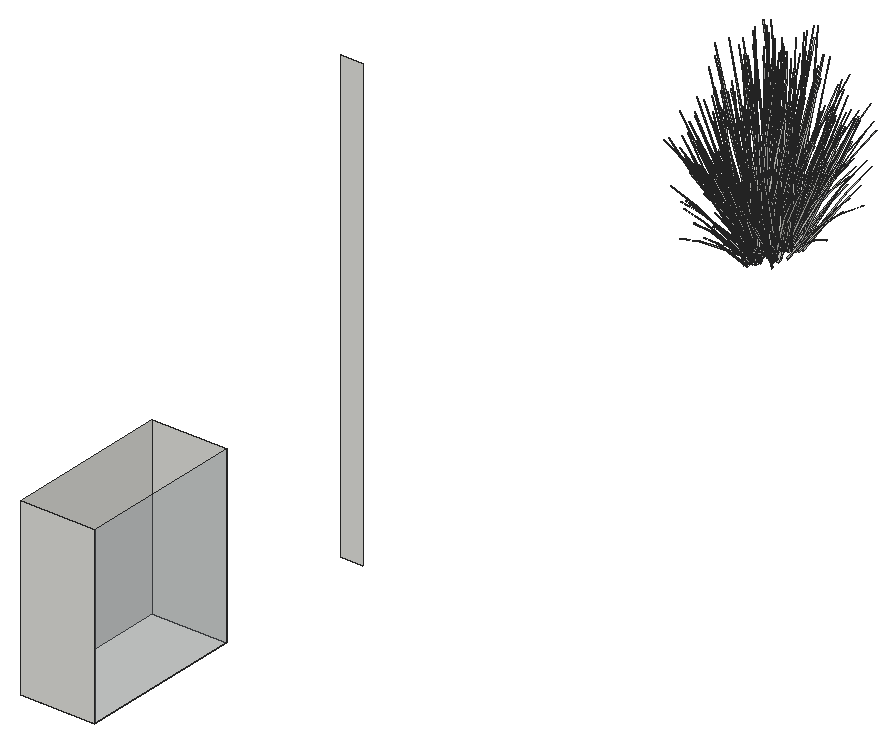
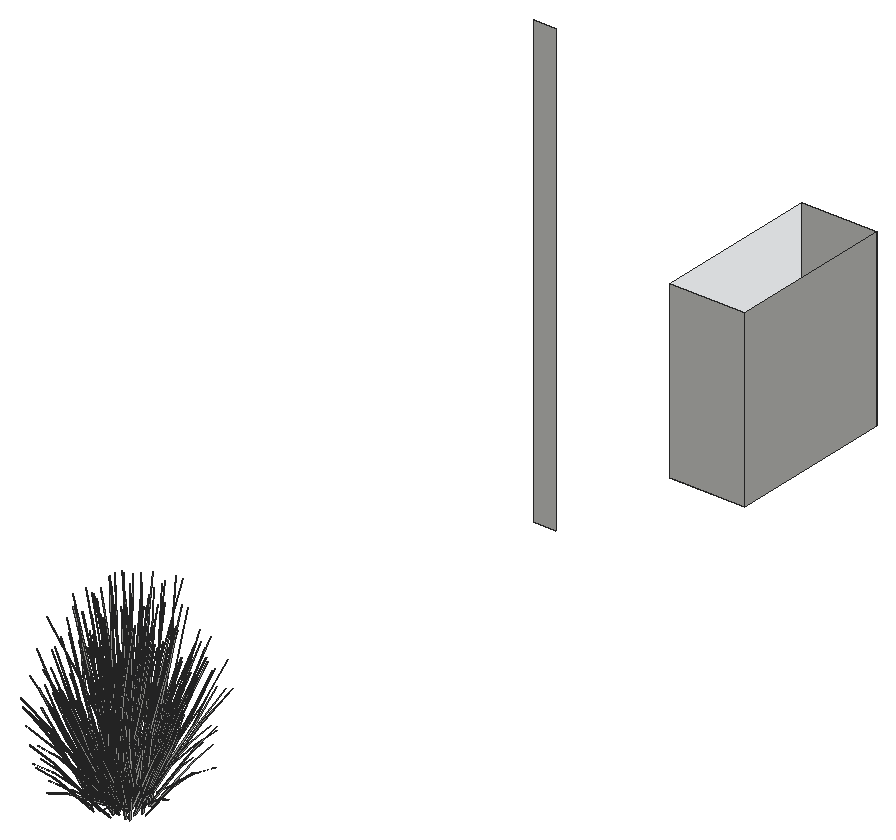
# SketchUp Ruby script. Lengths in inches.
U = 1.inch
M = Sketchup.active_model
def pt(a) = Geom::Point3d.new(a.map { |v| v * U })
def face(e, loops, mat)
  f = e.add_face(loops[0].map { |a| pt(a) })
  loops[1..].each { |l| e.add_face(l.map { |a| pt(a) }).erase! }
  f.material = f.back_material = mat if mat
  f
end
# faces: each face lists its corners as indices into pts; further lists are holes
def faces(e, pts, list, mat = nil) = list.each { |f| face(e, (f[0].is_a?(Array) ? f : [f]).map { |l| l.map { |i| pts[i] } }, mat) }
# xy, xz, yz: faces in a plane at the given z, y or x. An outline is a flat list of corners, or four numbers for a rectangle; further outlines are holes
def ring(l) = l.size == 4 ? [[l[0], l[1]], [l[2], l[1]], [l[2], l[3]], [l[0], l[3]]] : l.each_slice(2).to_a
def flat(e, list, mat, &to3) = list.each { |f| face(e, (f[0].is_a?(Array) ? f : [f]).map { |l| ring(l).map { |u, v| to3.(u, v) } }, mat) }
def xy(e, z, list, mat = nil) = flat(e, list, mat) { |x, y| [x, y, z] }
def xz(e, y, list, mat = nil) = flat(e, list, mat) { |x, z| [x, y, z] }
def yz(e, x, list, mat = nil) = flat(e, list, mat) { |y, z| [x, y, z] }
def lines(e, pts, list) = list.each { |a, b| e.add_line(pt(pts[a]), pt(pts[b])) }
# prism: a flat outline (further loops are holes) pulled along v
def prism(e, loops, v, mat = nil)
  f = face(e, loops, mat); d = Geom::Vector3d.new(v.map { |x| x * U })
  f.pushpull(f.normal.samedirection?(d) ? d.length : -d.length)
end
def box(e, o, s, mat = nil) = prism(e, [[o, [o[0] + s[0], o[1], o[2]], [o[0] + s[0], o[1] + s[1], o[2]], [o[0], o[1] + s[1], o[2]]]], [0, 0, s[2]], mat)
def at(x, y, z, deg = 0) = Geom::Transformation.translation(pt([x, y, z])) * Geom::Transformation.rotation(ORIGIN, Z_AXIS, deg.degrees)
def axes(o, x, y, z) = Geom::Transformation.new([*x, 0, *y, 0, *z, 0, *pt(o).to_a, 1])
def part(name) = M.definitions.add(name)
# library, detail: a bought-in or finely detailed component or shape, given as its bounding box
def library(name, o, s) = part(name).tap { |d| box(d.entities, o, s) }
def detail(e, o, s) = box(e.add_group.entities, o, s)
def put(e, d, t, mat = nil) = e.add_instance(d, t).tap { |i| i.material = mat if mat }
def group(e, t, mat = nil) = e.add_group.tap { |g| g.transformation = t; g.material = mat if mat }.entities
root = M.entities
M.materials.add("Glass_Basic_01").color = [161, 173, 186]
M.materials["Glass_Basic_01"].alpha = 0.25
c1 = part("blade")
p = [[2.15,0.21,22],[0,0.17,0],[0.09,0.45,0],[2.18,0.31,22],[2.29,0.31,22],[0.38,0.45,0],
  [2.48,0.24,33],[2.49,0.24,33],[2.48,0.22,33]]
faces(c1.entities,p,[[0,1,2,3],[4,5,2,3],[6,3,4,7],[8,0,3,6]])
c2 = part("blade with seeds\#1")
put(c2.entities,c1,at(0,0,0))
xy(root,122,[[460.07,50,480,94]])
xz(root,50,[[460.07,122,480,168.38]])
xz(root,94,[[460.07,122,480,168.38]])
xz(root,132,[[480,126,486,246]])
yz(root,460.07,[[50,122,94,168.38]])
yz(root,480,[[50,122,94,168.38]],"Glass_Basic_01")
put(root,c2,axes([472.34,285.93,129.63],[-1.0019,0.47479,-0.62955],[-0.36083,-1.36768,-0.16523],[-0.33927,0.05248,1.38963]))
put(root,c2,axes([474.05,281.59,129.625],[0.89455,-0.42392,-0.62393],[0.32217,1.22114,-0.16376],[0.30292,-0.04686,1.37722]))
put(root,c2,axes([472.17,281.71,129.59],[0.16018,-1.20264,-0.5621],[0.98808,0.25378,-0.14753],[0.11973,-0.3589,1.24074]))
put(root,c2,axes([474.21,285.74,129.59],[-0.16018,1.20264,-0.5621],[-0.98808,-0.25378,-0.14753],[-0.11973,0.3589,1.24074]))
put(root,c2,axes([471.31,283.85,129.59],[-0.73437,-0.77871,-0.5621],[0.66591,-0.96736,-0.14753],[-0.18319,-0.31204,1.24074]))
put(root,c2,axes([475.07,283.6,129.59],[0.73437,0.77871,-0.5621],[-0.66591,0.96736,-0.14753],[0.18319,0.31204,1.24074]))
put(root,c2,axes([470.3,280.13,129.56],[0.48852,-1.08202,-0.44759],[0.87598,0.64674,0],[0.11126,-0.24644,1.41987]))
put(root,c2,axes([477.07,282.32,129.56],[0.48852,1.08202,-0.44759],[-0.87598,0.64674,0],[0.11126,0.24644,1.41987]))
put(root,c2,axes([472.2,288.72,129.56],[-0.97703,0,-0.44759],[0,-1.29348,0],[-0.22253,0,1.41987]))
put(root,c2,axes([476.08,287.32,129.56],[-0.48852,1.08202,-0.44759],[-0.87598,-0.64674,0],[-0.11126,0.24644,1.41987]))
put(root,c2,axes([469.3125,285.13,129.56],[-0.48852,-1.08202,-0.44759],[0.87598,-0.64674,0],[-0.11126,-0.24644,1.41987]))
put(root,c2,axes([474.18,278.72,129.56],[0.97703,0,-0.44759],[0,1.29348,0],[0.22253,0,1.41987]))
put(root,c2,axes([472.6,285.2,129.73],[-0.88038,-0.56093,-0.40331],[0.4237,-1.16553,0.1941],[-0.20294,0,1.29492]))
put(root,c2,axes([473.9,285.12,129.73],[-0.82007,0.69452,-0.40331],[-0.57748,-1.05199,0.1941],[-0.10147,0.22475,1.29492]))
put(root,c2,axes([472.48,282.33,129.73],[0.82007,-0.69452,-0.40331],[0.57748,1.05199,0.1941],[0.10147,-0.22475,1.29492]))
put(root,c2,axes([473.78,282.25,129.73],[0.88038,0.56093,-0.40331],[-0.4237,1.16553,0.1941],[0.20294,0,1.29492]))
put(root,c2,axes([474.49,283.64,129.73],[0.06031,1.25545,-0.40331],[-1.00118,0.11354,0.1941],[0.10147,0.22475,1.29492]))
put(root,c2,axes([469.7,284.88,129.57],[0.24175,-1.0786,-0.27926],[0.85134,0.27158,0.27926],[-0.09817,-0.21744,1.25283]))
put(root,c2,axes([474.16,279.28,129.57],[0.60959,0.80703,-0.27926],[-0.60959,0.80703,0.27926],[0.19635,0,1.25283]))
put(root,c2,axes([475.72,287.02,129.57],[-0.85134,0.27158,-0.27926],[-0.24175,-1.0786,0.27926],[-0.09817,0.21744,1.25283]))
put(root,c2,axes([476.68,282.57,129.57],[-0.24175,1.0786,-0.27926],[-0.85134,-0.27158,0.27926],[0.09817,0.21744,1.25283]))
put(root,c2,axes([470.66,280.43,129.57],[0.85134,-0.27158,-0.27926],[0.24175,1.0786,0.27926],[0.09817,-0.21744,1.25283]))
put(root,c2,axes([472.22,288.17,129.57],[-0.60959,-0.80703,-0.27926],[0.60959,-0.80703,0.27926],[-0.19635,0,1.25283]))
put(root,c2,axes([477.25,280.18,129.08],[-0.14106,-0.08423,1.5897],[-0.41543,-1.06044,-0.24285],[0.21501,-0.3215,0.27078]))
put(root,c2,axes([472.82,289.61,129.08],[0.15398,-0.02932,1.5897],[0.80412,0.59108,-0.24285],[-0.04053,0.41985,0.27078]))
put(root,c2,axes([467.6,284.33,129.08],[0.0352,0.19392,1.5897],[-0.39624,1.07238,-0.24285],[-0.33051,-0.01799,0.27078]))
put(root,c2,axes([477.22,285.14,129.08],[-0.05317,-0.18711,1.5897],[0.29263,-1.12549,-0.24285],[0.32981,-0.03291,0.27078]))
put(root,c2,axes([472.97,277.13,129.08],[-0.14833,0.06042,1.5897],[-0.86768,-0.41907,-0.24285],[-0.01248,-0.42273,0.27078]))
put(root,c2,axes([468.81,287.79,129.08],[0.12871,0.11199,1.5897],[0.2775,1.13173,-0.24285],[-0.25244,0.2734,0.27078]))
put(root,c2,axes([477.13,289.92,129.08],[0.09761,-0.15508,1.5897],[0.90442,-0.26295,-0.24285],[0.19286,0.3437,0.27078]))
put(root,c2,axes([469.28,279.58,129.08],[-0.07697,0.17304,1.5897],[-0.85991,0.44448,-0.24285],[-0.23336,-0.29985,0.27078]))
put(root,c2,axes([471.44,286.02,129.17],[0.39117,1.13797,1.16227],[-1.12236,0.3622,0.45161],[0.01867,-0.69878,1.32195]))
put(root,c2,axes([475.32,282.36,129.71],[-0.33151,-1.21377,-0.17307],[0.95493,-0.4265,0.00007],[-0.03664,-0.13398,1.56765]))
put(root,c2,axes([474.22,282.76,130.14],[1.11485,-0.13472,-0.26229],[0.06741,1.40314,-0.45076],[0.1485,0.24708,1.43974]))
put(root,c2,axes([473.05,282.11,130.14],[0.46619,-1.302,-0.26229],[0.98396,0.62692,-0.45076],[0.24158,-0.04092,1.43974]))
put(root,c2,axes([473.33,285.34,130.14],[-0.46619,1.302,-0.26229],[-0.98396,-0.62692,-0.45076],[-0.24158,0.04092,1.43974]))
put(root,c2,axes([472.17,284.69,130.14],[-1.11485,0.13472,-0.26229],[-0.06741,-1.40314,-0.45076],[-0.1485,-0.24708,1.43974]))
put(root,c2,axes([472.02,283.07,130.14],[-0.64866,-1.16728,-0.26229],[0.91655,-0.77622,-0.45076],[0.09308,-0.288,1.43974]))
put(root,c2,axes([474.36,284.375,130.14],[0.64866,1.16728,-0.26229],[-0.91655,0.77622,-0.45076],[-0.09308,0.288,1.43974]))
put(root,c2,axes([474.65,283.07,129.96],[-0.78639,1.12892,-0.2271],[-0.88305,-0.94994,0.49699],[0.09199,0.304,1.51643]))
put(root,c2,axes([474.37,285.02,129.94],[-1.15773,-0.30643,-0.21121],[0.20181,-1.4529,0.4622],[-0.15988,0.25387,1.41028]))
put(root,c2,axes([468.28,284.53,129.65],[0.56051,0.79893,-0.03509],[-0.61388,0.73204,-0.15911],[-0.17394,0.05154,0.52479]))
put(root,c2,axes([469.3,288.5,129.65],[0.7978,0.33351,-0.03509],[-0.24541,1.02647,-0.15911],[-0.13049,0.15585,0.52479]))
put(root,c2,axes([472.75,276.59,129.77],[-0.62476,0.71677,-0.05849],[-0.57245,-0.78502,-0.26518],[-0.0403,-0.22243,0.87466]))
put(root,c2,axes([473.58,277.94,129.52],[0.11725,0.74462,1.27635],[-0.9333,0.11852,0.07306],[-0.14126,-0.52153,0.72629]))
put(root,c2,axes([469.46,286.11,129.875],[-0.97904,0.72283,0],[-0.54599,-1.20931,-0.46523],[-0.12435,-0.27543,1.47583]))
put(root,c2,axes([476.67,286.66,129.875],[0.97904,0.72283,0],[-0.54599,1.20931,-0.46523],[-0.12435,0.27543,1.47583]))
put(root,c2,axes([476.92,281.34,129.875],[0.97904,-0.72283,0],[0.54599,1.20931,-0.46523],[0.12435,0.27543,1.47583]))
put(root,c2,axes([472.94,289.05,129.875],[0,1.44565,0],[-1.09198,0,-0.46523],[-0.24871,0,1.47583]))
put(root,c2,axes([475.47,283.13,129.8],[1.12244,-0.50265,-0.0542],[0.39331,1.43622,0],[0.0392,-0.01755,1.55211]))
put(root,c2,axes([469.71,280.79,129.88],[-0.97904,-0.72283,0],[0.54599,-1.20931,-0.46523],[0.12435,-0.27543,1.47583]))
put(root,c2,axes([473.4375,278.4,129.88],[0,-1.44565,0],[1.09198,0,-0.46523],[0.24871,0,1.47583]))
put(root,c2,axes([473.71,282.8,129.81],[-0.84094,1.07538,-0.05527],[-0.84146,-1.07603,0],[-0.02937,0.03755,1.58274]))
put(root,c2,axes([473.28,282.4375,129.8],[1.12994,0,-0.05082],[0,1.44565,0],[0.03551,0,1.61697]))
put(root,c2,axes([476.81,282.25,129.71],[-0.98246,0.71382,-0.04636],[-0.54599,-1.20931,0.46523],[0.09354,0.298,1.4751]))
put(root,c2,axes([474,278.98,129.72],[-0.00781,1.44494,-0.04486],[-1.09198,0,0.45022],[0.24858,0.04541,1.42752]))
put(root,c2,axes([472.66,287.93,129.84],[0.82143,1.07538,0.27726],[-0.81279,1.07603,-0.32897],[-0.23327,0.03755,1.48641]))
put(root,c2,axes([476.3,282.22,129.84],[0.31757,-1.44738,0.27726],[1.13512,0.3621,-0.32897],[0.14207,0.23956,1.48641]))
put(root,c2,axes([475.82,284.03,129.72],[-0.43865,1.16553,0],[-0.91144,-0.56093,0],[0,0,1.46678]))
put(root,c2,axes([475.44,283.77,129.72],[-0.84234,0.37722,0],[-0.29498,-1.07717,0],[0,0,1.39163]))
put(root,c2,axes([475.84,282.71,129.72],[0.43865,-1.16553,0],[0.91144,0.56093,0],[0,0,1.57718]))
put(root,c2,axes([472.83,283.17,129.72],[-1.1305,0,0],[0,-1.44565,0],[0,0,1.61777]))
put(root,c2,axes([473.09,282.18,129.73],[0,-1.29348,0],[1.0115,0,0],[0,0,1.60831]))
put(root,c2,axes([473.52,282.21,129.73],[0.63109,-0.80703,0],[0.63109,0.80703,0],[0,0,1.52591]))
put(root,c2,axes([473.8125,284.85,129.87],[0.20585,-1.46124,0.41247],[1.16261,0.29738,0.16186],[-0.11226,0.21355,1.43206]))
put(root,c2,axes([472.12,283.85,129.87],[0.88667,0.95859,0.41247],[-0.7827,1.13884,0.16186],[-0.08849,-0.2311,1.43206]))
put(root,c2,axes([472.74,284.97,129.87],[1.09253,-0.50265,0.41247],[0.37991,1.43622,0.16186],[-0.20075,-0.01755,1.43206]))
put(root,c2,axes([472.57,282.6,129.88],[-0.20585,1.46124,0.44352],[-1.16261,-0.29738,0.17404],[0.11226,-0.21355,1.53985]))
put(root,c2,axes([474.43,282.5,130.1],[0.58702,-0.85413,0.13053],[0.66228,0.71246,-0.37274],[0.08953,0.19831,1.14258]))
put(root,c2,axes([471.74,282.96,130.1],[-0.87196,-0.22303,0.13053],[0.15136,-1.08968,-0.37274],[0.08953,-0.19831,1.14258]))
put(root,c2,axes([472.98,281.74,130.1],[-0.28493,-1.07717,0.13053],[0.81364,-0.37722,-0.37274],[0.17907,0,1.14258]))
put(root,c2,axes([474.64,284.49,130.1],[0.87196,0.22303,0.13053],[-0.15136,1.08968,-0.37274],[-0.08953,0.19831,1.14258]))
put(root,c2,axes([477.35,287.72,130.28],[-0.17302,-1.05027,0.05866],[0.69705,-0.24145,-0.77802],[0.35285,0.06658,0.69739]))
put(root,c2,axes([470.99,288.8,130.07],[0.27202,-0.22572,1.28914],[0.7394,0.52014,-0.27724],[-0.17673,0.53408,0.55117]))
put(root,c2,axes([478.09,287.98,130.07],[-0.15413,-0.36483,1.28914],[0.46474,-0.90077,-0.27724],[0.40213,0.2681,0.55117]))
put(root,c2,axes([475.91,282.68,130.07],[-0.32388,-0.0204,1.28914],[-0.36177,-0.97496,-0.27724],[0.38765,-0.30097,0.55117]))
put(root,c2,axes([468.67,281.875,130.07],[0.19776,0.32863,1.28914],[-0.34614,0.98419,-0.27724],[-0.43048,-0.18244,0.55117]))
put(root,c2,axes([471,278.71,130.07],[-0.02894,0.41302,1.28914],[-0.77632,0.42312,-0.27724],[-0.21961,-0.50739,0.55117]))
put(root,c2,axes([468.3,286.96,130.07],[0.31962,0.07001,1.28914],[0.26756,1.02347,-0.27724],[-0.41311,0.23924,0.55117]))
put(root,c2,axes([474.96,277.73,130.07],[-0.2403,0.27843,1.28914],[-0.79492,-0.36227,-0.27724],[0.10768,-0.56334,0.55117]))
put(root,c2,axes([474.96,290.35,130.07],[0.08021,-0.40179,1.28914],[0.81924,-0.25896,-0.27724],[0.15335,0.54576,0.55117]))
put(root,c2,axes([473.11,288.17,129.97],[0.97703,0,0.44759],[0,1.29348,0],[-0.22253,0,1.41987]))
put(root,c2,axes([470.22,281.41,129.97],[-0.48852,1.08202,0.44759],[-0.87598,-0.64674,0],[0.11126,-0.24644,1.41987]))
put(root,c2,axes([473.27,279.28,129.97],[-0.97703,0,0.44759],[0,-1.29348,0],[0.22253,0,1.41987]))
put(root,c2,axes([476.24,281.59,129.97],[-0.48852,-1.08202,0.44759],[0.87598,-0.64674,0],[0.11126,0.24644,1.41987]))
put(root,c2,axes([476.16,286.04,129.97],[0.48852,-1.08202,0.44759],[0.87598,0.64674,0],[-0.11126,0.24644,1.41987]))
put(root,c2,axes([473.04,284.51,129.93],[0.47355,-1.30265,0.21694],[0.98396,0.62692,0.45076],[-0.22682,0,1.44726]))
put(root,c2,axes([470.71,281.82,129.97],[0.25932,1.24233,0.15904],[-0.96507,0.30677,0.3163],[0.14061,-0.1108,1.44604]))
put(root,c2,axes([473.24,280.03,129.97],[-0.71168,0.90835,0.15904],[-0.69029,-0.91538,0.3163],[0.14534,0.10032,1.44604]))
put(root,c2,axes([470.66,285.51,129.97],[0.971,0.33398,0.15904],[-0.27478,1.22215,0.3163],[-0.00473,-0.21112,1.44604]))
put(root,c2,axes([475.72,281.94,129.97],[-0.971,-0.33398,0.15904],[0.27478,-1.22215,0.3163],[0.00473,0.21112,1.44604]))
put(root,c2,axes([475.67,285.63,129.97],[-0.25932,-1.24233,0.15904],[0.96507,-0.30677,0.3163],[-0.14061,0.1108,1.44604]))
put(root,c2,axes([472.78,282.22,130.1875],[-0.88038,-0.56093,0.40331],[0.4237,-1.16553,-0.1941],[0.20294,0,1.29492]))
put(root,c2,axes([472.38,284.93,130.1875],[0.06031,1.25545,0.40331],[-1.00118,0.11354,-0.1941],[-0.10147,-0.22475,1.29492]))
put(root,c2,axes([471.97,283.43,130.1875],[-0.82007,0.69452,0.40331],[-0.57748,-1.05199,-0.1941],[0.10147,-0.22475,1.29492]))
put(root,c2,axes([473.6,285.23,130.1875],[0.88038,0.56093,0.40331],[-0.4237,1.16553,-0.1941],[-0.20294,0,1.29492]))
put(root,c2,axes([474,282.52,130.1875],[-0.06031,-1.25545,0.40331],[1.00118,-0.11354,-0.1941],[0.10147,0.22475,1.29492]))
put(root,c2,axes([477.48,280.26,130.14],[-0.03064,0.74138,0.9471],[-0.6508,-0.48961,0.52291],[0.23122,-0.29288,0.74292]))
put(root,c2,axes([471.81,290.15,130.23],[-0.06991,-0.73811,1.03545],[0.616,0.4682,0.76078],[-0.09241,0.36475,0.22807]))
put(root,c2,axes([476.21,280.37,130.23],[-0.28093,0.65095,1.03545],[-0.28545,-0.84053,0.76078],[0.2418,-0.22671,0.22807]))
put(root,c2,axes([476.67,291.19,130.23],[-0.44281,-0.48182,1.03545],[0.70101,-0.19012,0.76078],[0.12552,0.34819,0.22807]))
put(root,c2,axes([473.9,276.4,130.23],[0.1613,0.71432,1.03545],[-0.66662,-0.33623,0.76078],[0.04561,-0.37895,0.22807]))
put(root,c2,axes([467.78,287.32,130.23],[0.34005,-0.60308,1.03545],[0.20441,0.87829,0.76078],[-0.26134,0.18792,0.22807]))
put(root,c2,axes([478.61,287.11,130.23],[-0.58095,0.02992,1.03545],[0.41436,-0.74764,0.76078],[0.2769,0.14704,0.22807]))
put(root,c2,axes([469.57,278.23,130.23],[0.49736,0.38508,1.03545],[-0.66822,0.331,0.76078],[-0.16744,-0.31805,0.22807]))
put(root,c2,axes([467.1,283.09,130.23],[0.56973,-0.14831,1.03545],[-0.31555,0.82274,0.76078],[-0.29172,-0.08853,0.22807]))
put(root,c2,axes([473.04,281.95,130.3],[-0.91991,0.03158,1.27354],[0.23846,-1.42935,0.53923],[0.50337,0.33806,1.20213]))
put(root,c2,axes([469.58,285.86,132.23],[-0.47225,0.98582,-0.64046],[-0.82754,-0.7006,0.07729],[-0.28197,0.35717,0.906]))
put(root,c2,axes([476.84,284.79,132.23],[0.79444,-0.5518,-0.64046],[0.44274,1.13586,0.07729],[0.38385,-0.12903,0.906]))
put(root,c2,axes([470.75,287.87,132.23],[-0.02352,1.1557,-0.64046],[-0.99061,-0.07762,0.07729],[-0.10454,0.48961,0.906]))
put(root,c2,axes([471.71,279.58,132.23],[-0.77091,-0.6039,-0.64046],[0.54787,-1.05824,0.07729],[-0.27931,-0.36058,0.906]))
put(root,c2,axes([473.65,279.3,132.23],[-0.4315,-1.0159,-0.64046],[0.88824,-0.56616,0.07729],[-0.1009,-0.49086,0.906]))
put(root,c2,axes([470.14,281.08,132.23],[-0.90375,-0.03008,-0.64046],[0.0607,-1.26677,0.07729],[-0.38287,-0.13368,0.906]))
put(root,c2,axes([475.45,280.29,132.23],[0.02352,-1.1557,-0.64046],[0.99061,0.07762,0.07729],[0.10454,-0.48961,0.906]))
put(root,c2,axes([469.36,283.375,132.23],[-0.79444,0.5518,-0.64046],[-0.44274,-1.13586,0.07729],[-0.38385,0.12903,0.906]))
put(root,c2,axes([477,284.37,131.96],[0.24493,-1.13649,-0.46065],[0.83975,0.38955,-0.35681],[0.33809,-0.10421,0.88141]))
put(root,c2,axes([469.84,281.33,131.96],[-0.65648,0.82762,-0.46065],[-0.57493,-0.87428,-0.35681],[-0.33354,-0.12593,0.88141]))
put(root,c2,axes([469.61,286.32,131.96],[0.23225,1.14083,-0.46065],[-0.87956,0.19957,-0.35681],[-0.25205,0.30642,0.88141]))
put(root,c2,axes([473.33,279.09,131.96],[-0.88873,-0.31321,-0.46065],[0.30463,-1.07385,-0.35681],[-0.08149,-0.43235,0.88141]))
put(root,c2,axes([470.95,288.25,131.96],[0.6472,0.83949,-0.46065],[-0.68369,0.73521,-0.35681],[-0.09847,0.42653,0.88141]))
put(root,c2,axes([474.85,288.55,131.96],[0.89213,-0.297,-0.46065],[0.15606,1.12475,-0.35681],[0.23962,0.32232,0.88141]))
put(root,c2,axes([472.87,289.07,131.96],[0.88873,0.31321,-0.46065],[-0.30463,1.07385,-0.35681],[0.08149,0.43235,0.88141]))
put(root,c2,axes([469.2,283.79,131.96],[-0.24493,1.13649,-0.46065],[-0.83975,-0.38955,-0.35681],[-0.33809,0.10421,0.88141]))
put(root,c2,axes([471.35,279.61,131.96],[-0.89213,0.297,-0.46065],[-0.15606,-1.12475,-0.35681],[-0.23962,-0.32232,0.88141]))
put(root,c2,axes([476.59,281.84,131.96],[-0.23225,-1.14083,-0.46065],[0.87956,-0.19957,-0.35681],[0.25205,-0.30642,0.88141]))
put(root,c2,axes([472.33,286.8,130.75],[-0.14134,-0.32863,1.5962],[0.98684,-0.11332,0.12492],[0.13095,0.71181,0.57049]))
put(root,c2,axes([476.0625,287.08,132.55],[0.90375,0.03008,-0.71091],[-0.0607,1.26677,0.08579],[0.38287,0.13368,1.00565]))
put(root,c2,axes([476.36,286.83,132.25],[0.65648,-0.82762,-0.51132],[0.57493,0.87428,-0.39606],[0.33354,0.12593,0.97836]))
put(root,c2,axes([477.34,287.51,130.77],[-0.50438,-0.0254,1.3914],[0.26641,-1.14247,0.19228],[0.53755,0.09899,0.65702]))
put(root,c2,axes([474.93,283.5,130.73],[0.39398,-0.99907,1.36359],[0.84877,0.97875,0.53923],[-0.50305,0.4384,1.14314]))
put(root,c2,axes([475.86,279.59,131.82],[0.61172,-0.65782,-0.31925],[0.57907,0.75112,0.41216],[0.08811,-0.38163,0.78863]))
put(root,c2,axes([472.47,289.73,131.82],[-0.27256,0.96081,-0.31925],[-0.79518,-0.28024,0.41216],[0.07291,0.38684,0.78863]))
put(root,c2,axes([474.76,289.375,131.82],[0.13963,1.00636,-0.31925],[-0.79822,0.26574,0.41216],[0.2144,0.28839,0.78863]))
put(root,c2,axes([473.73,278.43,131.82],[0.27256,-0.96081,-0.31925],[0.79518,0.28024,0.41216],[-0.07291,-0.38684,0.78863]))
put(root,c2,axes([468.96,286.2,131.82],[-0.78697,0.17856,-0.31925],[-0.2078,-1.02074,0.41216],[-0.22552,0.27417,0.78863]))
put(root,c2,axes([476.61,287.6,131.82],[0.51441,0.78225,-0.31925],[-0.58738,0.7405,0.41216],[0.29843,0.11267,0.78863]))
put(root,c2,axes([471.44,278.78,131.82],[-0.13963,-1.00636,-0.31925],[0.79822,-0.26574,0.41216],[-0.2144,-0.28839,0.78863]))
put(root,c2,axes([477.52,284.89,131.82],[0.75135,0.34854,-0.31925],[-0.21915,1.01686,0.41216],[0.30251,-0.09324,0.78863]))
put(root,c2,axes([469.59,280.56,131.82],[-0.51441,-0.78225,-0.31925],[0.58738,-0.7405,0.41216],[-0.29843,-0.11267,0.78863]))
put(root,c2,axes([468.68,283.27,131.82],[-0.75135,-0.34854,-0.31925],[0.21915,-1.01686,0.41216],[-0.30251,0.09324,0.78863]))
put(root,c2,axes([470.34,288.57,131.82],[-0.61172,0.65782,-0.31925],[-0.57907,-0.75112,0.41216],[-0.08811,0.38163,0.78863]))
put(root,c2,axes([475.95,277.64,131.28],[-0.82131,0.22128,-0.03148],[-0.18882,-1.04586,-0.14272],[0.05207,-0.2184,0.47074]))
put(root,c2,axes([474.29,281.96,131.23],[-0.16834,0.42944,1.54493],[-0.70619,-0.88871,0.12492],[0.31858,-0.5539,0.66044]))
put(root,c2,axes([469.68,282.5,131.23],[0.33582,0.21526,1.54493],[-0.69497,0.90306,0.12492],[-0.43315,-0.40739,0.66044]))
put(root,c2,axes([472.75,281.05,131.23],[0.02213,0.47954,1.54493],[-0.95907,-0.31812,0.12492],[0.05932,-0.68338,0.66044]))
put(root,c2,axes([475.27,283.73,131.23],[-0.31369,0.26428,1.54493],[-0.26409,-1.22118,0.12492],[0.49247,-0.276,0.66044]))
put(root,c2,axes([475.42,285.88,131.23],[-0.375,0.0283,1.54493],[0.24877,-1.22643,0.12492],[0.53441,0.07586,0.66044]))
put(root,c2,axes([474.71,287.85,131.23],[-0.33582,-0.21526,1.54493],[0.69497,-0.90306,0.12492],[0.43315,0.40739,0.66044]))
put(root,c2,axes([473.33,289.11,131.23],[-0.20666,-0.40114,1.54493],[0.95496,-0.33772,0.12492],[0.21583,0.62976,0.66044]))
put(root,c2,axes([473.97,287.64,131.23],[-0.3002,-0.28876,1.54493],[0.81031,-0.72911,0.12492],[0.36902,0.50009,0.66044]))
put(root,c2,axes([469.125,286.63,131.23],[0.31369,-0.26428,1.54493],[0.26409,1.22118,0.12492],[-0.49247,0.276,0.66044]))
put(root,c2,axes([470.1,288.4,131.23],[0.16834,-0.42944,1.54493],[0.70619,0.88871,0.12492],[-0.31858,0.5539,0.66044]))
put(root,c2,axes([471.64,289.3,131.23],[-0.02213,-0.47954,1.54493],[0.95907,0.31812,0.12492],[-0.05932,0.68338,0.66044]))
put(root,c2,axes([475.93,280.35,132.28],[-0.99362,-0.0619,-0.10962],[0.02716,-1.17208,-0.60845],[0.06902,-0.45141,0.92453]))
put(root,c2,axes([472.11,289.12,132.28],[0.88471,-0.5817,-0.10962],[0.43476,1.03242,-0.60845],[0.11673,0.43507,0.92453]))
put(root,c2,axes([470.18,280.47,132.28],[-0.04841,1.27062,-0.10962],[-0.91657,-0.03473,-0.60845],[-0.353,-0.08826,0.92453]))
put(root,c2,axes([474.09,279.04,132.28],[-0.88471,0.5817,-0.10962],[-0.43476,-1.03242,-0.60845],[-0.11673,-0.43507,0.92453]))
put(root,c2,axes([477.04,285.34,132.28],[-0.45489,-1.13134,-0.10962],[0.80735,-0.55596,-0.60845],[0.34022,-0.14927,0.92453]))
put(root,c2,axes([470.27,287.8125,132.28],[0.99362,0.0619,-0.10962],[-0.02716,1.17208,-0.60845],[-0.06902,0.45141,0.92453]))
put(root,c2,axes([477.01,282.65,132.28],[-0.8363,-0.68892,-0.10962],[0.4818,-0.99769,-0.60845],[0.23628,-0.3468,0.92453]))
put(root,c2,axes([474.21,289.08,132.28],[0.53874,-1.06944,-0.10962],[0.78019,0.61612,-0.60845],[0.2712,0.30214,0.92453]))
put(root,c2,axes([469.16,282.82,132.28],[0.45489,1.13134,-0.10962],[-0.80735,0.55596,-0.60845],[-0.34022,0.14927,0.92453]))
put(root,c2,axes([471.99,279.08,132.28],[-0.53874,1.06944,-0.10962],[-0.78019,-0.61612,-0.60845],[-0.2712,-0.30214,0.92453]))
put(root,c2,axes([472.07,281.875,131.77],[-0.50765,0.99901,1.24659],[-0.79039,-1.05487,0.53787],[0.47632,-0.32232,1.20495]))
put(root,c2,axes([473,290.33,131.99],[0.12685,0.18879,1.57709],[0.92682,-0.01606,-0.24942],[0.12053,0.43275,0.12648]))
put(root,c2,axes([472.7,275.88,131.99],[-0.14882,-0.16043,1.57709],[-0.91289,0.20534,-0.24942],[-0.17308,-0.40254,0.12648]))
put(root,c2,axes([475.33,279.33,131.99],[-0.01652,-0.24801,1.57709],[-0.75906,-0.68026,-0.24942],[0.1002,-0.44114,0.12648]))
put(root,c2,axes([468.72,279.3125,131.99],[-0.19445,0.01116,1.57709],[-0.562,0.94258,-0.24942],[-0.34067,-0.14573,0.12648]))
put(root,c2,axes([476.46,290.3,131.99],[0.19335,0.02874,1.57709],[0.67262,-0.81555,-0.24942],[0.31807,0.21351,0.12648]))
put(root,c2,axes([478.85,285.61,131.99],[0.15733,-0.14655,1.57709],[0.06181,-1.18266,-0.24942],[0.34698,-0.11893,0.12648]))
put(root,c2,axes([467.05,284.61,131.99],[-0.13699,0.17683,1.57709],[0.08685,1.18009,-0.24942],[-0.32765,0.18834,0.12648]))
put(root,c2,axes([468.55,288.48,131.99],[-0.0069,0.24875,1.57709],[0.68965,0.79195,-0.24942],[-0.14092,0.42256,0.12648]))
put(root,c2,axes([469.14,289.4375,131.98],[0.0975,-0.08571,1.59908],[0.87648,0.41319,-0.1511],[0.00634,0.41846,0.28298]))
put(root,c2,axes([466.6,285.82,131.98],[0.11711,0.02157,1.59908],[0.42502,1.06376,-0.1511],[-0.21726,0.31303,0.28298]))
put(root,c2,axes([477.7,283.56,131.98],[-0.11829,-0.00342,1.59908],[-0.52187,-0.99076,-0.1511],[0.18628,-0.34414,0.28298]))
put(root,c2,axes([473.93,292.43,131.98],[0.0262,-0.14755,1.59908],[0.86326,-0.45644,-0.1511],[0.22658,0.30203,0.28298]))
put(root,c2,axes([471.75,276.45,131.98],[-0.00742,0.151,1.59908],[-0.79509,0.62706,-0.1511],[-0.26143,-0.25182,0.28298]))
put(root,c2,axes([476.72,276.73,131.98],[-0.08553,0.10454,1.59908],[-0.91687,-0.22868,-0.1511],[-0.05858,-0.41178,0.28298]))
put(root,c2,axes([478.4375,290.39,131.98],[-0.05899,-0.13116,1.59908],[0.39237,-1.08407,-0.1511],[0.32669,0.02548,0.28298]))
put(root,c2,axes([468.03,279.5625,131.98],[0.07463,0.11741,1.59908],[-0.25178,1.15035,-0.1511],[-0.32567,0.04164,0.28298]))
put(root,c2,axes([476.02,287.69,132.6],[0.04841,-1.27062,-0.12168],[0.91657,0.03473,-0.67538],[0.353,0.08826,1.02623]))
put(root,c2,axes([468.82,285.52,132.63],[0.93666,0.77159,-0.12278],[-0.53962,1.11741,-0.68147],[-0.26463,0.38842,1.03548]))
put(root,c2,axes([468.86,283.14,132],[0.25543,-1.1392,0.43274],[0.83975,0.38955,0.35681],[-0.33023,0.06846,0.89544]))
put(root,c2,axes([475.85,279.85,132],[0.64379,0.85247,0.43274],[-0.68369,0.73521,0.35681],[0.11875,-0.39995,0.89544]))
put(root,c2,axes([473.83,278.66,132],[0.89085,0.32663,0.43274],[-0.30463,1.07385,0.35681],[-0.05354,-0.4223,0.89544]))
put(root,c2,axes([474.59,289.24,132],[-0.89921,0.28673,0.43274],[-0.15606,-1.12475,0.35681],[0.21148,0.33149,0.89544]))
put(root,c2,axes([476.41,287.6,132],[-0.66663,0.82326,0.43274],[-0.57493,-0.87428,0.35681],[0.31276,0.15186,0.89544]))
put(root,c2,axes([469.79,280.56,132],[0.66663,-0.82326,0.43274],[0.57493,0.87428,0.35681],[-0.31276,-0.15186,0.89544]))
put(root,c2,axes([472.37,289.5,132],[-0.89085,-0.32663,0.43274],[0.30463,-1.07385,0.35681],[0.05354,0.4223,0.89544]))
put(root,c2,axes([471.61,278.91,132],[0.89921,-0.28673,0.43274],[0.15606,1.12475,0.35681],[-0.21148,-0.33149,0.89544]))
put(root,c2,axes([477.14,282.18,132],[0.22422,1.14989,0.43274],[-0.87956,0.19957,0.35681],[0.25922,-0.27044,0.89544]))
put(root,c2,axes([468.89,285.76,132],[-0.62066,-0.52545,0.05797],[0.36135,-0.74826,0.45634],[-0.19899,0.24191,0.69585]))
put(root,c2,axes([477.41,285.32,132],[0.33205,0.8519,0.05797],[-0.60551,0.41697,0.45634],[0.26692,-0.08227,0.69585]))
put(root,c2,axes([471.79,278.69,132],[0.4109,-0.79368,0.05797],[0.58514,0.46209,0.45634],[-0.18917,-0.25446,0.69585]))
put(root,c2,axes([474.07,278.57,132],[0.66618,-0.42462,0.05797],[0.32607,0.77431,0.45634],[-0.06434,-0.34133,0.69585]))
put(root,c2,axes([470.11,288.23,132],[-0.74296,-0.05822,0.05797],[0.02037,-0.87906,0.45634],[-0.07774,0.33673,0.69585]))
put(root,c2,axes([469.86,280.25,132],[0.04552,-0.95007,0.05797],[0.68742,0.02605,0.45634],[-0.26332,-0.09941,0.69585]))
put(root,c2,axes([476.09,279.93,132],[0.74296,0.05822,0.05797],[-0.02037,0.87906,0.45634],[0.07774,-0.33673,0.69585]))
put(root,c2,axes([474.41,289.47,132],[-0.4109,0.79368,0.05797],[-0.58514,-0.46209,0.45634],[0.18917,0.25446,0.69585]))
put(root,c2,axes([468.79,282.84,132],[-0.33205,-0.8519,0.05797],[0.60551,-0.41697,0.45634],[-0.26692,0.08227,0.69585]))
put(root,c2,axes([472.13,289.59,132],[-0.66618,0.42462,0.05797],[-0.32607,-0.77431,0.45634],[0.06434,0.34133,0.69585]))
put(root,c2,axes([477.3125,282.4,132],[0.62066,0.52545,0.05797],[-0.36135,0.74826,0.45634],[0.19899,-0.24191,0.69585]))
put(root,c2,axes([476.34,287.9,132],[-0.04552,0.95007,0.05797],[-0.68742,-0.02605,0.45634],[0.26332,0.09941,0.69585]))
put(root,c2,axes([476.72,285,132.29],[-0.75135,-0.34854,0.31925],[0.21915,-1.01686,-0.41216],[0.30251,-0.09324,0.78863]))
put(root,c2,axes([469.48,283.16,132.29],[0.75135,0.34854,0.31925],[-0.21915,1.01686,-0.41216],[-0.30251,0.09324,0.78863]))
put(root,c2,axes([475.54,280.53,132.29],[-0.61172,0.65782,0.31925],[-0.57907,-0.75112,-0.41216],[0.08811,-0.38163,0.78863]))
put(root,c2,axes([473.82,279.45,132.29],[-0.27256,0.96081,0.31925],[-0.79518,-0.28024,-0.41216],[-0.07291,-0.38684,0.78863]))
put(root,c2,axes([470.66,287.63,132.29],[0.61172,-0.65782,0.31925],[0.57907,0.75112,-0.41216],[-0.08811,0.38163,0.78863]))
put(root,c2,axes([475.88,287.2,132.29],[-0.51441,-0.78225,0.31925],[0.58738,-0.7405,-0.41216],[0.29843,0.11267,0.78863]))
put(root,c2,axes([474.29,288.55,132.29],[-0.13963,-1.00636,0.31925],[0.79822,-0.26574,-0.41216],[0.2144,0.28839,0.78863]))
put(root,c2,axes([476.6,282.5625,132.29],[-0.78697,0.17856,0.31925],[-0.2078,-1.02074,-0.41216],[0.22552,-0.27417,0.78863]))
put(root,c2,axes([471.91,279.61,132.29],[0.13963,1.00636,0.31925],[-0.79822,0.26574,-0.41216],[-0.2144,-0.28839,0.78863]))
put(root,c2,axes([472.38,288.71,132.29],[0.27256,-0.96081,0.31925],[0.79518,0.28024,-0.41216],[0.07291,0.38684,0.78863]))
put(root,c2,axes([470.32,280.96,132.29],[0.51441,0.78225,0.31925],[-0.58738,0.7405,-0.41216],[-0.29843,-0.11267,0.78863]))
put(root,c2,axes([469.6,285.6,132.29],[0.78697,-0.17856,0.31925],[0.2078,1.02074,-0.41216],[-0.22552,0.27417,0.78863]))
put(root,c2,axes([477.34,285.02,132.3],[-0.25543,1.1392,0.48034],[-0.83975,-0.38955,0.39606],[0.33023,-0.06846,0.99394]))
put(root,c2,axes([470.11,288.66,132.33],[-0.72104,-0.95477,0.48466],[0.76573,-0.82343,0.39963],[-0.133,0.44794,1.00289]))
put(root,c2,axes([468.67,286.06,132.33],[-0.25113,-1.28788,0.48466],[0.9851,-0.22351,0.39963],[-0.29033,0.30289,1.00289]))
put(root,c2,axes([479.4,283.63,132.83],[-0.56051,-0.79893,-0.05849],[0.61388,-0.73204,-0.26518],[0.17394,-0.05154,0.87466]))
put(root,c2,axes([476.55,290.84,132.83],[0.2608,-1.0202,-0.05849],[0.8027,0.31383,-0.26518],[0.12187,0.16686,0.87466]))
